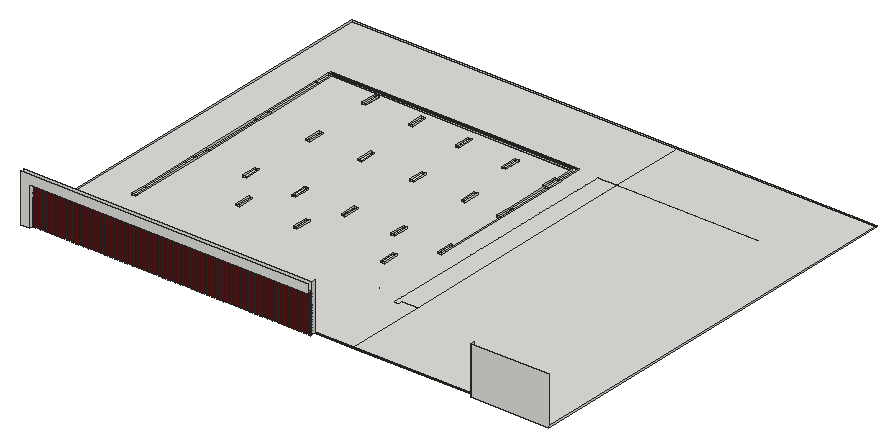
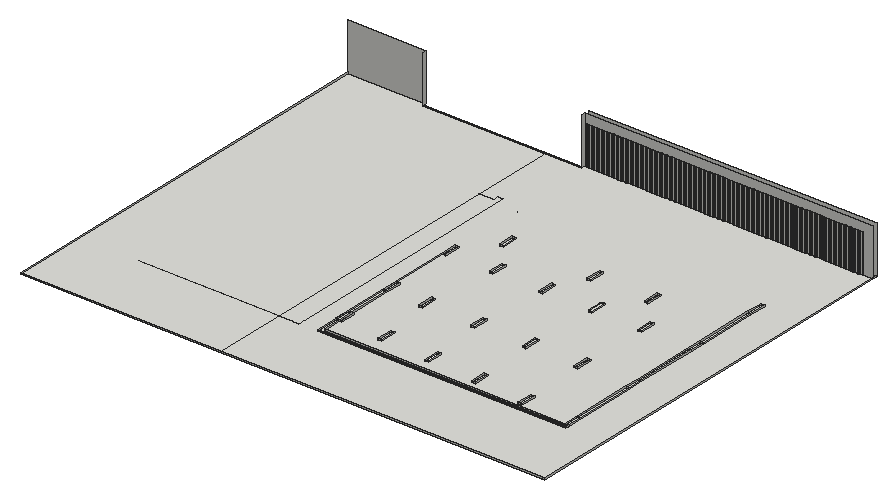
# SketchUp Ruby script. Lengths in inches.
U = 1.inch
M = Sketchup.active_model
def pt(a) = Geom::Point3d.new(a.map { |v| v * U })
def face(e, loops, mat)
  f = e.add_face(loops[0].map { |a| pt(a) })
  loops[1..].each { |l| e.add_face(l.map { |a| pt(a) }).erase! }
  f.material = f.back_material = mat if mat
  f
end
# faces: each face lists its corners as indices into pts; further lists are holes
def faces(e, pts, list, mat = nil) = list.each { |f| face(e, (f[0].is_a?(Array) ? f : [f]).map { |l| l.map { |i| pts[i] } }, mat) }
# xy, xz, yz: faces in a plane at the given z, y or x. An outline is a flat list of corners, or four numbers for a rectangle; further outlines are holes
def ring(l) = l.size == 4 ? [[l[0], l[1]], [l[2], l[1]], [l[2], l[3]], [l[0], l[3]]] : l.each_slice(2).to_a
def flat(e, list, mat, &to3) = list.each { |f| face(e, (f[0].is_a?(Array) ? f : [f]).map { |l| ring(l).map { |u, v| to3.(u, v) } }, mat) }
def xy(e, z, list, mat = nil) = flat(e, list, mat) { |x, y| [x, y, z] }
def xz(e, y, list, mat = nil) = flat(e, list, mat) { |x, z| [x, y, z] }
def yz(e, x, list, mat = nil) = flat(e, list, mat) { |y, z| [x, y, z] }
def lines(e, pts, list) = list.each { |a, b| e.add_line(pt(pts[a]), pt(pts[b])) }
# prism: a flat outline (further loops are holes) pulled along v
def prism(e, loops, v, mat = nil)
  f = face(e, loops, mat); d = Geom::Vector3d.new(v.map { |x| x * U })
  f.pushpull(f.normal.samedirection?(d) ? d.length : -d.length)
end
def box(e, o, s, mat = nil) = prism(e, [[o, [o[0] + s[0], o[1], o[2]], [o[0] + s[0], o[1] + s[1], o[2]], [o[0], o[1] + s[1], o[2]]]], [0, 0, s[2]], mat)
def at(x, y, z, deg = 0) = Geom::Transformation.translation(pt([x, y, z])) * Geom::Transformation.rotation(ORIGIN, Z_AXIS, deg.degrees)
def axes(o, x, y, z) = Geom::Transformation.new([*x, 0, *y, 0, *z, 0, *pt(o).to_a, 1])
def part(name) = M.definitions.add(name)
# library, detail: a bought-in or finely detailed component or shape, given as its bounding box
def library(name, o, s) = part(name).tap { |d| box(d.entities, o, s) }
def detail(e, o, s) = box(e.add_group.entities, o, s)
def put(e, d, t, mat = nil) = e.add_instance(d, t).tap { |i| i.material = mat if mat }
def group(e, t, mat = nil) = e.add_group.tap { |g| g.transformation = t; g.material = mat if mat }.entities
root = M.entities
M.materials.add("[0022_Maroon]").color = [128, 0, 0]
xy(root,-3,[[0,0,22.65,12],[22.65,9,29.85,12],[34.34,9,41.53,12],[46.03,9,53.22,12],[57.71,9,64.91,12],
  [69.4,9,76.6,12],[81.09,9,88.28,12],[92.78,9,99.97,12],[104.46,9,111.66,12],[116.15,9,123.35,12],
  [127.84,9,135.03,12],[139.53,9,146.72,12],[151.21,9,158.41,12],[162.9,9,170.1,12],[174.59,9,181.78,12],
  [186.28,9,193.47,12],[197.96,9,205.16,12],[209.65,9,216.85,12],[221.34,9,228.53,12],[233.03,9,240.22,12],
  [244.71,9,251.91,12],[256.4,9,263.6,12],[268.09,9,275.28,12],[279.78,9,286.97,12],[291.46,9,298.66,12],
  [303.15,9,310.35,12],[314.84,9,322.03,12],[326.53,9,333.72,12],[338.21,9,345.41,12],[349.9,9,357.1,12],
  [361.59,9,368.78,12],[373.28,9,380.47,12],[384.96,9,392.16,12],[396.65,9,403.85,12],[408.34,9,415.53,12],
  [420.03,9,427.22,12],[431.71,9,438.91,12],[443.4,9,450.6,12],[455.09,9,462.28,12],[466.78,9,473.97,12],
  [478.46,9,485.66,12],[490.15,9,497.35,12],[501.84,9,509.03,12],[513.53,9,520.72,12],[525.21,9,532.41,12],
  [536.9,9,544.1,12],[548.59,9,555.78,12],[560.28,9,567.47,12],[571.96,9,579.16,12],[583.65,9,590.85,12],
  [595.34,9,602.53,12],[607.03,9,614.22,12],[618.9,9,626.1,12],[630.78,9,637.97,12],[642.65,9,649.85,12],
  [654.53,9,661.72,12],[666.4,9,673.6,12],[678.28,9,685.47,12],[690.15,9,695.72,12],[[0,12,0,1001.99,785.81,1001.99,785.81,821.88,737.47,821.88,737.47,207.2,748.75,207.2,748.75,218.45,785.81,218.45,785.81,21,695.72,21,695.72,12],[92.9,222.09,101.9,222.09,101.9,813.09,683.9,813.09,683.9,767.49,678.47,767.49,678.47,729.63,683.9,729.63,683.9,623.66,683.76,623.66,683.76,585.81,692.76,585.81,692.76,623.66,683.9,623.66,683.9,729.63,692.9,729.63,692.9,444.51,684.15,444.51,684.15,406.65,693.15,406.65,693.15,444.51,692.9,444.51,692.9,822.09,92.9,822.09],[684.07,729.63,693.07,767.49],[212.28,406.65,221.28,444.51],[331.65,406.65,340.65,444.51],[451.03,406.65,460.03,444.51],[570.4,406.65,579.4,444.51],[218.09,591.22,227.09,629.07],[343.28,591.22,352.28,629.07],[468.47,591.22,477.47,629.07],[593.65,591.22,602.65,629.07],[333.32,757.32,342.32,795.18],[453.53,748.09,462.53,785.95],[573.74,738.86,582.74,776.72],[271.23,312.53,280.23,350.39],[410.36,312.53,419.36,350.39],[621.3,312.53,630.3,350.39],[213.11,766.55,222.11,804.4],[684.15,406.65,692.9,444.51]],
  [1078.65,12,1078.65,21,785.81,21,785.81,1001.99,1267.9,1001.99,1267.9,12],[737.47,207.2,737.47,821.88,785.81,821.88,785.81,218.45,748.75,218.45,748.75,207.2],[92.9,222.09,101.9,259.95],[92.9,259.95,101.9,406.65],[271.23,312.53,280.23,350.39],
  [410.36,312.53,419.36,350.39],[621.3,312.53,630.3,350.39],[92.9,406.65,101.9,444.51],[212.28,406.65,221.28,444.51],[331.65,406.65,340.65,444.51],
  [451.03,406.65,460.03,444.51],[570.4,406.65,579.4,444.51],[684.15,406.65,692.9,444.51],[92.9,444.51,101.9,591.22],[683.9,585.81,692.76,623.66],
  [92.9,591.22,101.9,629.07],[218.09,591.22,227.09,629.07],[343.28,591.22,352.28,629.07],[468.47,591.22,477.47,629.07],[593.65,591.22,602.65,629.07],
  [92.9,629.07,101.9,775.78],[678.47,729.63,684.07,767.49],[684.07,729.63,692.9,767.49],[573.74,738.86,582.74,776.72],[333.32,757.32,342.32,795.18],
  [213.11,766.55,222.11,804.4],[683.9,767.49,683.9,813.09,101.9,813.09,101.9,813.63,92.9,813.63,92.9,822.09,692.9,822.09,692.9,767.49],[92.9,775.78,101.9,813.63]])
xy(root,-0.625,[[331.65,406.65,340.65,444.51]])
xz(root,0,[[0,-3,22.65,-3,22.65,90.43,695.72,90.43,695.72,112.5625,0,112.5625]])
xz(root,9,[[22.65,-3,29.85,90.43],[34.34,-3,41.53,90.43],[46.03,-3,53.22,90.43],[57.71,-3,64.91,90.43],[69.4,-3,76.6,90.43],
  [81.09,-3,88.28,90.43],[92.78,-3,99.97,90.43],[104.46,-3,111.66,90.43],[116.15,-3,123.35,90.43],[127.84,-3,135.03,90.43],
  [139.53,-3,146.72,90.43],[151.21,-3,158.41,90.43],[162.9,-3,170.1,90.43],[174.59,-3,181.78,90.43],[186.28,-3,193.47,90.43],
  [197.96,-3,205.16,90.43],[209.65,-3,216.85,90.43],[221.34,-3,228.53,90.43],[233.03,-3,240.22,90.43],[244.71,-3,251.91,90.43],
  [256.4,-3,263.6,90.43],[268.09,-3,275.28,90.43],[279.78,-3,286.97,90.43],[291.46,-3,298.66,90.43],[303.15,-3,310.35,90.43],
  [314.84,-3,322.03,90.43],[326.53,-3,333.72,90.43],[338.21,-3,345.41,90.43],[349.9,-3,357.1,90.43],[361.59,-3,368.78,90.43],
  [373.28,-3,380.47,90.43],[384.96,-3,392.16,90.43],[396.65,-3,403.85,90.43],[408.34,-3,415.53,90.43],[420.03,-3,427.22,90.43],
  [431.71,-3,438.91,90.43],[443.4,-3,450.6,90.43],[455.09,-3,462.28,90.43],[466.78,-3,473.97,90.43],[478.46,-3,485.66,90.43],
  [490.15,-3,497.35,90.43],[501.84,-3,509.03,90.43],[513.53,-3,520.72,90.43],[525.21,-3,532.41,90.43],[536.9,-3,544.1,90.43],
  [548.59,-3,555.78,90.43],[560.28,-3,567.47,90.43],[571.96,-3,579.16,90.43],[583.65,-3,590.85,90.43],[595.34,-3,602.53,90.43],
  [607.03,-3,614.22,90.43],[618.9,-3,626.1,90.43],[630.78,-3,637.97,90.43],[642.65,-3,649.85,90.43],[654.53,-3,661.72,90.43],
  [666.4,-3,673.6,90.43],[678.28,-3,685.47,90.43],[690.15,-3,695.72,90.43]],"[0022_Maroon]")
xz(root,12,[[0,-3,0,112.5625,695.72,112.5625,695.72,90.43,22.65,90.43,22.65,-3],[22.65,-3,29.85,90.43],[34.34,-3,41.53,90.43],[46.03,-3,53.22,90.43],[57.71,-3,64.91,90.43],
  [69.4,-3,76.6,90.43],[81.09,-3,88.28,90.43],[92.78,-3,99.97,90.43],[104.46,-3,111.66,90.43],[116.15,-3,123.35,90.43],
  [127.84,-3,135.03,90.43],[139.53,-3,146.72,90.43],[151.21,-3,158.41,90.43],[162.9,-3,170.1,90.43],[174.59,-3,181.78,90.43],
  [186.28,-3,193.47,90.43],[197.96,-3,205.16,90.43],[209.65,-3,216.85,90.43],[221.34,-3,228.53,90.43],[233.03,-3,240.22,90.43],
  [244.71,-3,251.91,90.43],[256.4,-3,263.6,90.43],[268.09,-3,275.28,90.43],[279.78,-3,286.97,90.43],[291.46,-3,298.66,90.43],
  [303.15,-3,310.35,90.43],[314.84,-3,322.03,90.43],[326.53,-3,333.72,90.43],[338.21,-3,345.41,90.43],[349.9,-3,357.1,90.43],
  [361.59,-3,368.78,90.43],[373.28,-3,380.47,90.43],[384.96,-3,392.16,90.43],[396.65,-3,403.85,90.43],[408.34,-3,415.53,90.43],
  [420.03,-3,427.22,90.43],[431.71,-3,438.91,90.43],[443.4,-3,450.6,90.43],[455.09,-3,462.28,90.43],[466.78,-3,473.97,90.43],
  [478.46,-3,485.66,90.43],[490.15,-3,497.35,90.43],[501.84,-3,509.03,90.43],[513.53,-3,520.72,90.43],[525.21,-3,532.41,90.43],
  [536.9,-3,544.1,90.43],[548.59,-3,555.78,90.43],[560.28,-3,567.47,90.43],[571.96,-3,579.16,90.43],[583.65,-3,590.85,90.43],
  [595.34,-3,602.53,90.43],[607.03,-3,614.22,90.43],[618.9,-3,626.1,90.43],[630.78,-3,637.97,90.43],[642.65,-3,649.85,90.43],
  [654.53,-3,661.72,90.43],[666.4,-3,673.6,90.43],[678.28,-3,685.47,90.43],[690.15,-3,695.72,90.43],[1078.65,-3,1267.9,112.5625]])
xz(root,12,[[29.85,-3,34.34,90.43],[41.53,-3,46.03,90.43],[53.22,-3,57.71,90.43],[64.91,-3,69.4,90.43],[76.6,-3,81.09,90.43],
  [88.28,-3,92.78,90.43],[99.97,-3,104.46,90.43],[111.66,-3,116.15,90.43],[123.35,-3,127.84,90.43],[135.03,-3,139.53,90.43],
  [146.72,-3,151.21,90.43],[158.41,-3,162.9,90.43],[170.1,-3,174.59,90.43],[181.78,-3,186.28,90.43],[193.47,-3,197.96,90.43],
  [205.16,-3,209.65,90.43],[216.85,-3,221.34,90.43],[228.53,-3,233.03,90.43],[240.22,-3,244.71,90.43],[251.91,-3,256.4,90.43],
  [263.6,-3,268.09,90.43],[275.28,-3,279.78,90.43],[286.97,-3,291.46,90.43],[298.66,-3,303.15,90.43],[310.35,-3,314.84,90.43],
  [322.03,-3,326.53,90.43],[333.72,-3,338.21,90.43],[345.41,-3,349.9,90.43],[357.1,-3,361.59,90.43],[368.78,-3,373.28,90.43],
  [380.47,-3,384.96,90.43],[392.16,-3,396.65,90.43],[403.85,-3,408.34,90.43],[415.53,-3,420.03,90.43],[427.22,-3,431.71,90.43],
  [438.91,-3,443.4,90.43],[450.6,-3,455.09,90.43],[462.28,-3,466.78,90.43],[473.97,-3,478.46,90.43],[485.66,-3,490.15,90.43],
  [497.35,-3,501.84,90.43],[509.03,-3,513.53,90.43],[520.72,-3,525.21,90.43],[532.41,-3,536.9,90.43],[544.1,-3,548.59,90.43],
  [555.78,-3,560.28,90.43],[567.47,-3,571.96,90.43],[579.16,-3,583.65,90.43],[590.85,-3,595.34,90.43],[602.53,-3,607.03,90.43],
  [614.22,-3,618.9,90.43],[626.1,-3,630.78,90.43],[637.97,-3,642.65,90.43],[649.85,-3,654.53,90.43],[661.72,-3,666.4,90.43],
  [673.6,-3,678.28,90.43],[685.47,-3,690.15,90.43]],"[0022_Maroon]")
xz(root,21,[[695.72,-3,1078.65,0]])
xz(root,222.09,[[92.9,-3,101.9,0]])
xz(root,312.53,[[271.23,-3,280.23,0],[410.36,-3,419.36,0],[621.3,-3,630.3,0]])
xz(root,350.39,[[271.23,-3,280.23,0],[410.36,-3,419.36,0],[621.3,-3,630.3,0]])
xz(root,406.65,[[92.9,-3,101.9,0],[212.28,-3,221.28,0],[331.65,-3,340.65,-0.625],[451.03,-3,460.03,0],[570.4,-3,579.4,0],
  [684.15,-3,692.9,0],[692.9,-3,693.15,0],[331.65,-0.625,340.65,0]])
xz(root,444.51,[[92.9,-3,101.9,0],[212.28,-3,221.28,0],[331.65,-3,340.65,-0.625],[451.03,-3,460.03,0],[570.4,-3,579.4,0],
  [684.15,-3,692.9,0],[692.9,-3,693.15,0],[331.65,-0.625,340.65,0]])
xz(root,585.81,[[683.76,-3,683.9,0],[683.9,-3,692.76,0]])
xz(root,591.22,[[92.9,-3,101.9,0],[218.09,-3,227.09,0],[343.28,-3,352.28,0],[468.47,-3,477.47,0],[593.65,-3,602.65,0]])
xz(root,623.66,[[683.76,-3,683.9,0],[683.9,-3,692.76,0]])
xz(root,629.07,[[92.9,-3,101.9,0],[218.09,-3,227.09,0],[343.28,-3,352.28,0],[468.47,-3,477.47,0],[593.65,-3,602.65,0]])
xz(root,729.63,[[678.47,-3,683.9,0],[683.9,-3,684.07,0],[684.07,-3,692.9,0],[692.9,-3,693.07,0]])
xz(root,738.86,[[573.74,-3,582.74,0]])
xz(root,748.09,[[453.53,-3,462.53,0]])
xz(root,757.32,[[333.32,-3,342.32,0]])
xz(root,766.55,[[213.11,-3,222.11,0]])
xz(root,767.49,[[678.47,-3,683.9,0],[683.9,-3,684.07,0],[684.07,-3,692.9,0],[692.9,-3,693.07,0]])
xz(root,775.78,[[92.9,-3,101.9,0]])
xz(root,776.72,[[573.74,-3,582.74,0]])
xz(root,785.95,[[453.53,-3,462.53,0]])
xz(root,795.18,[[333.32,-3,342.32,0]])
xz(root,804.4,[[213.11,-3,222.11,0]])
xz(root,813.09,[[101.9,-3,683.9,0]])
xz(root,813.63,[[92.9,-3,101.9,0]])
xz(root,822.09,[[92.9,-3,692.9,0]])
xz(root,1001.99,[[0,-3,1267.9,0]])
yz(root,0,[[0,-3,12,0],[12,-3,1001.99,0]])
yz(root,22.65,[[0,-3,9,90.43],[9,-3,12,90.43]])
yz(root,29.85,[[9,-3,12,90.43]],"[0022_Maroon]")
yz(root,34.34,[[9,-3,12,90.43]])
yz(root,41.53,[[9,-3,12,90.43]],"[0022_Maroon]")
yz(root,46.03,[[9,-3,12,90.43]])
yz(root,53.22,[[9,-3,12,90.43]],"[0022_Maroon]")
yz(root,57.71,[[9,-3,12,90.43]])
yz(root,64.91,[[9,-3,12,90.43]],"[0022_Maroon]")
yz(root,69.4,[[9,-3,12,90.43]])
yz(root,76.6,[[9,-3,12,90.43]],"[0022_Maroon]")
yz(root,81.09,[[9,-3,12,90.43]])
yz(root,88.28,[[9,-3,12,90.43]],"[0022_Maroon]")
yz(root,92.78,[[9,-3,12,90.43]])
yz(root,92.9,[[222.09,-3,259.95,0],[259.95,-3,406.65,0],[406.65,-3,444.51,0],[444.51,-3,591.22,0],[591.22,-3,629.07,0],
  [629.07,-3,775.78,0],[775.78,-3,813.63,0],[813.63,-3,822.09,0]])
yz(root,99.97,[[9,-3,12,90.43]],"[0022_Maroon]")
yz(root,101.9,[[222.09,-3,231.09,0],[231.09,-3,259.95,0],[259.95,-3,406.65,0],[406.65,-3,444.51,0],[444.51,-3,591.22,0],
  [591.22,-3,629.07,0],[629.07,-3,775.78,0],[775.78,-3,813.09,0],[813.09,-3,813.63,0]])
yz(root,104.46,[[9,-3,12,90.43]])
yz(root,111.66,[[9,-3,12,90.43]],"[0022_Maroon]")
yz(root,116.15,[[9,-3,12,90.43]])
yz(root,123.35,[[9,-3,12,90.43]],"[0022_Maroon]")
yz(root,127.84,[[9,-3,12,90.43]])
yz(root,135.03,[[9,-3,12,90.43]],"[0022_Maroon]")
yz(root,139.53,[[9,-3,12,90.43]])
yz(root,146.72,[[9,-3,12,90.43]],"[0022_Maroon]")
yz(root,151.21,[[9,-3,12,90.43]])
yz(root,158.41,[[9,-3,12,90.43]],"[0022_Maroon]")
yz(root,162.9,[[9,-3,12,90.43]])
yz(root,170.1,[[9,-3,12,90.43]],"[0022_Maroon]")
yz(root,174.59,[[9,-3,12,90.43]])
yz(root,181.78,[[9,-3,12,90.43]],"[0022_Maroon]")
yz(root,186.28,[[9,-3,12,90.43]])
yz(root,193.47,[[9,-3,12,90.43]],"[0022_Maroon]")
yz(root,197.96,[[9,-3,12,90.43]])
yz(root,205.16,[[9,-3,12,90.43]],"[0022_Maroon]")
yz(root,209.65,[[9,-3,12,90.43]])
yz(root,212.28,[[406.65,-3,444.51,0]])
yz(root,213.11,[[766.55,-3,804.4,0]])
yz(root,216.85,[[9,-3,12,90.43]],"[0022_Maroon]")
yz(root,218.09,[[591.22,-3,629.07,0]])
yz(root,221.28,[[406.65,-3,444.51,0]])
yz(root,221.34,[[9,-3,12,90.43]])
yz(root,222.11,[[766.55,-3,803.86,0],[803.86,-3,804.4,0]])
yz(root,227.09,[[591.22,-3,629.07,0]])
yz(root,228.53,[[9,-3,12,90.43]],"[0022_Maroon]")
yz(root,233.03,[[9,-3,12,90.43]])
yz(root,240.22,[[9,-3,12,90.43]],"[0022_Maroon]")
yz(root,244.71,[[9,-3,12,90.43]])
yz(root,251.91,[[9,-3,12,90.43]],"[0022_Maroon]")
yz(root,256.4,[[9,-3,12,90.43]])
yz(root,263.6,[[9,-3,12,90.43]],"[0022_Maroon]")
yz(root,268.09,[[9,-3,12,90.43]])
yz(root,271.23,[[312.53,-3,350.39,0]])
yz(root,275.28,[[9,-3,12,90.43]],"[0022_Maroon]")
yz(root,279.78,[[9,-3,12,90.43]])
yz(root,280.23,[[312.53,-3,350.39,0]])
yz(root,286.97,[[9,-3,12,90.43]],"[0022_Maroon]")
yz(root,291.46,[[9,-3,12,90.43]])
yz(root,298.66,[[9,-3,12,90.43]],"[0022_Maroon]")
yz(root,303.15,[[9,-3,12,90.43]])
yz(root,310.35,[[9,-3,12,90.43]],"[0022_Maroon]")
yz(root,314.84,[[9,-3,12,90.43]])
yz(root,322.03,[[9,-3,12,90.43]],"[0022_Maroon]")
yz(root,326.53,[[9,-3,12,90.43]])
yz(root,331.65,[[406.65,-3,444.51,-0.625],[406.65,-0.625,444.51,0]])
yz(root,333.32,[[757.32,-3,795.18,0]])
yz(root,333.72,[[9,-3,12,90.43]],"[0022_Maroon]")
yz(root,338.21,[[9,-3,12,90.43]])
yz(root,340.65,[[406.65,-3,444.51,-0.625],[406.65,-0.625,444.51,0]])
yz(root,342.32,[[757.32,-3,794.63,0],[794.63,-3,795.18,0]])
yz(root,343.28,[[591.22,-3,629.07,0]])
yz(root,345.41,[[9,-3,12,90.43]],"[0022_Maroon]")
yz(root,349.9,[[9,-3,12,90.43]])
yz(root,352.28,[[591.22,-3,629.07,0]])
yz(root,357.1,[[9,-3,12,90.43]],"[0022_Maroon]")
yz(root,361.59,[[9,-3,12,90.43]])
yz(root,368.78,[[9,-3,12,90.43]],"[0022_Maroon]")
yz(root,373.28,[[9,-3,12,90.43]])
yz(root,380.47,[[9,-3,12,90.43]],"[0022_Maroon]")
yz(root,384.96,[[9,-3,12,90.43]])
yz(root,392.16,[[9,-3,12,90.43]],"[0022_Maroon]")
yz(root,396.65,[[9,-3,12,90.43]],"[0022_Maroon]")
yz(root,403.85,[[9,-3,12,90.43]],"[0022_Maroon]")
yz(root,408.34,[[9,-3,12,90.43]])
yz(root,410.36,[[312.53,-3,350.39,0]])
yz(root,415.53,[[9,-3,12,90.43]],"[0022_Maroon]")
yz(root,419.36,[[312.53,-3,350.39,0]])
yz(root,420.03,[[9,-3,12,90.43]])
yz(root,427.22,[[9,-3,12,90.43]],"[0022_Maroon]")
yz(root,431.71,[[9,-3,12,90.43]])
yz(root,438.91,[[9,-3,12,90.43]],"[0022_Maroon]")
yz(root,443.4,[[9,-3,12,90.43]])
yz(root,450.6,[[9,-3,12,90.43]],"[0022_Maroon]")
yz(root,451.03,[[406.65,-3,444.51,0]])
yz(root,453.53,[[748.09,-3,785.95,0]])
yz(root,455.09,[[9,-3,12,90.43]])
yz(root,460.03,[[406.65,-3,444.51,0]])
yz(root,462.28,[[9,-3,12,90.43]],"[0022_Maroon]")
yz(root,462.53,[[748.09,-3,785.4,0],[785.4,-3,785.95,0]])
yz(root,466.78,[[9,-3,12,90.43]])
yz(root,468.47,[[591.22,-3,629.07,0]])
yz(root,473.97,[[9,-3,12,90.43]],"[0022_Maroon]")
yz(root,477.47,[[591.22,-3,629.07,0]])
yz(root,478.46,[[9,-3,12,90.43]])
yz(root,485.66,[[9,-3,12,90.43]],"[0022_Maroon]")
yz(root,490.15,[[9,-3,12,90.43]])
yz(root,497.35,[[9,-3,12,90.43]],"[0022_Maroon]")
yz(root,501.84,[[9,-3,12,90.43]])
yz(root,509.03,[[9,-3,12,90.43]],"[0022_Maroon]")
yz(root,513.53,[[9,-3,12,90.43]])
yz(root,520.72,[[9,-3,12,90.43]],"[0022_Maroon]")
yz(root,525.21,[[9,-3,12,90.43]])
yz(root,532.41,[[9,-3,12,90.43]],"[0022_Maroon]")
yz(root,536.9,[[9,-3,12,90.43]])
yz(root,544.1,[[9,-3,12,90.43]],"[0022_Maroon]")
yz(root,548.59,[[9,-3,12,90.43]])
yz(root,555.78,[[9,-3,12,90.43]],"[0022_Maroon]")
yz(root,560.28,[[9,-3,12,90.43]])
yz(root,567.47,[[9,-3,12,90.43]],"[0022_Maroon]")
yz(root,570.4,[[406.65,-3,444.51,0]])
yz(root,571.96,[[9,-3,12,90.43]])
yz(root,573.74,[[738.86,-3,776.72,0]])
yz(root,579.16,[[9,-3,12,90.43]],"[0022_Maroon]")
yz(root,579.4,[[406.65,-3,444.51,0]])
yz(root,582.74,[[738.86,-3,776.18,0],[776.18,-3,776.72,0]])
yz(root,583.65,[[9,-3,12,90.43]])
yz(root,590.85,[[9,-3,12,90.43]],"[0022_Maroon]")
yz(root,593.65,[[591.22,-3,629.07,0]])
yz(root,595.34,[[9,-3,12,90.43]])
yz(root,602.53,[[9,-3,12,90.43]],"[0022_Maroon]")
yz(root,602.65,[[591.22,-3,629.07,0]])
yz(root,607.03,[[9,-3,12,90.43]])
yz(root,614.22,[[9,-3,12,90.43]],"[0022_Maroon]")
yz(root,618.9,[[9,-3,12,90.43]])
yz(root,621.3,[[312.53,-3,350.39,0]])
yz(root,626.1,[[9,-3,12,90.43]],"[0022_Maroon]")
yz(root,630.3,[[312.53,-3,350.39,0]])
yz(root,630.78,[[9,-3,12,90.43]])
yz(root,637.97,[[9,-3,12,90.43]],"[0022_Maroon]")
yz(root,642.65,[[9,-3,12,90.43]])
yz(root,649.85,[[9,-3,12,90.43]],"[0022_Maroon]")
yz(root,654.53,[[9,-3,12,90.43]])
yz(root,661.72,[[9,-3,12,90.43]],"[0022_Maroon]")
yz(root,666.4,[[9,-3,12,90.43]])
yz(root,673.6,[[9,-3,12,90.43]],"[0022_Maroon]")
yz(root,678.28,[[9,-3,12,90.43]])
yz(root,678.47,[[729.63,-3,767.49,0]])
yz(root,683.76,[[585.81,-3,623.66,0]])
yz(root,683.9,[[585.81,-3,623.66,0],[623.66,-3,729.63,0],[767.49,-3,813.09,0]])
yz(root,684.07,[[729.63,-3,767.49,0]])
yz(root,684.15,[[406.65,-3,444.51,0]])
yz(root,685.47,[[9,-3,12,90.43]],"[0022_Maroon]")
yz(root,690.15,[[9,-3,12,90.43]])
yz(root,692.76,[[585.81,-3,623.66,0]])
yz(root,692.9,[[406.65,-3,444.51,0],[444.51,-3,729.63,0],[729.63,-3,767.49,0],[767.49,-3,822.09,0]])
yz(root,693.07,[[729.63,-3,738.63,0],[738.63,-3,766.95,0],[766.95,-3,767.49,0]])
yz(root,693.15,[[406.65,-3,415.65,0],[415.65,-3,444.51,0]])
yz(root,695.72,[[12,-3,21,112.5625]])
yz(root,695.72,[[9,-3,12,90.43]],"[0022_Maroon]")
yz(root,1078.65,[[12,-3,21,112.5625]])
yz(root,1267.9,[[12,-3,1001.99,0]])
p = [[683.9,231.09,0],[683.9,231.09,-3],[785.81,821.88,-3],[1125.97,821.88,-3]]
lines(root,p,[[0,1],[2,3]])
